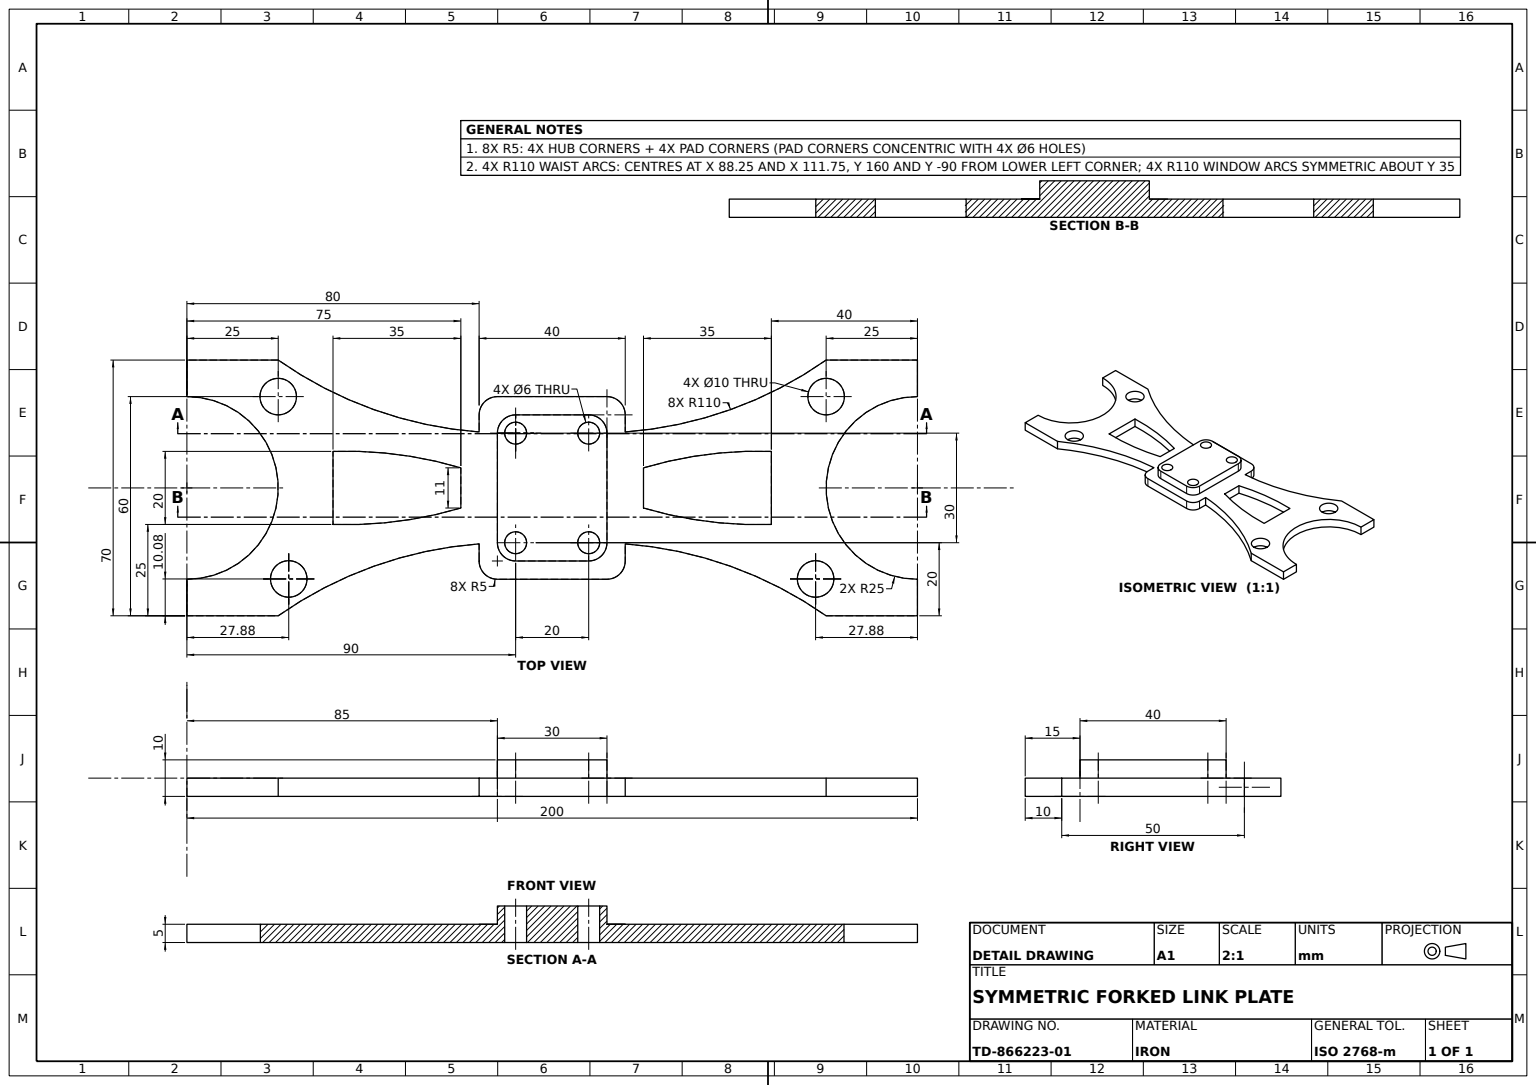
solid
v1 (100,35,-5)
v2 (75,35,-5)
e1 v1 v2 LINE
v3 (75,35,0)
e2 v3 v2 LINE
v4 (100,35,0)
e3 v4 v3 LINE
e4 v4 v1 LINE
face PLANE(AX(P(-100,35,0),D(0,1,0),D(1,0,0))) [e1 -e2 -e3 e4]
v5 (-20,15.309477,0)
v6 (-20,20,0)
e5 v5 v6 LINE
v7 (-20,20,-5)
e6 v6 v7 LINE
v8 (-20,15.309477,-5)
e7 v8 v7 LINE
e8 v5 v8 LINE
face PLANE(AX(P(-20,15.309477,0),D(-1,0,0),D(0,1,0))) [e5 e6 -e7 -e8]
v9 (20,20,-5)
v10 (20,15.309477,-5)
e9 v9 v10 LINE
v11 (20,20,0)
e10 v11 v9 LINE
v12 (20,15.309477,0)
e11 v11 v12 LINE
e12 v12 v10 LINE
face PLANE(AX(P(20,-15.309477,0),D(1,0,0),D(0,-1,0))) [-e9 -e10 e11 e12]
v13 (-15,-15,0)
v14 (-15,15,0)
e13 v13 v14 LINE
v15 (-15,-15,5)
e14 v13 v15 LINE
v16 (-15,15,5)
e15 v15 v16 LINE
e16 v14 v16 LINE
face PLANE(AX(P(-15,-20,0),D(1,0,0),D(0,1,0))) rev [-e13 e14 e15 -e16]
v17 (-100,-25,0)
v18 (-100,-35,0)
e17 v17 v18 LINE
v19 (-100,-25,-5)
e18 v17 v19 LINE
v20 (-100,-35,-5)
e19 v19 v20 LINE
e20 v18 v20 LINE
face PLANE(AX(P(-100,25,0),D(-1,0,0),D(0,1,0))) [-e17 e18 e19 -e20]
v21 (-20,-15.309477,-5)
v22 (-75,-35,-5)
e21 v21 v22 CIRCLE(AX(P(-11.754447,-125,-5),D(0,0,1),D(1,0,0)),110)
v23 (-20,-15.309477,0)
e22 v23 v21 LINE
v24 (-75,-35,0)
e23 v23 v24 CIRCLE(AX(P(-11.754447,-125,0),D(0,0,1),D(1,0,0)),110)
e24 v24 v22 LINE
face CYL(AX(P(-11.754447,-125,-2.5),D(0,0,1),D(1,0,0)),110) rev [-e21 -e22 e23 e24]
v25 (15,-25,-5)
v26 (-15,-25,-5)
e25 v25 v26 LINE
v27 (15,-25,0)
e26 v27 v25 LINE
v28 (-15,-25,0)
e27 v27 v28 LINE
e28 v28 v26 LINE
face PLANE(AX(P(20,-25,0),D(0,-1,0),D(-1,0,0))) [-e25 -e26 e27 e28]
v29 (75,-35,0)
v30 (75,-35,-5)
e29 v29 v30 LINE
v31 (20,-15.309477,0)
e30 v29 v31 CIRCLE(AX(P(11.754447,-125,0),D(0,0,1),D(1,0,0)),110)
v32 (20,-15.309477,-5)
e31 v31 v32 LINE
e32 v30 v32 CIRCLE(AX(P(11.754447,-125,-5),D(0,0,1),D(1,0,0)),110)
face CYL(AX(P(11.754447,-125,-2.5),D(0,0,1),D(1,0,0)),110) rev [-e29 e30 e31 -e32]
v33 (-10,-20,0)
v34 (-10,-20,5)
e33 v33 v34 LINE
e34 v15 v34 CIRCLE(AX(P(-10,-15,5),D(0,0,1),D(1,0,0)),5)
e35 v13 v33 CIRCLE(AX(P(-10,-15,0),D(0,0,1),D(1,0,0)),5)
face CYL(AX(P(-10,-15,2.5),D(0,0,1),D(0,-1,0)),5) [e33 -e34 -e14 e35]
v35 (60,10,-5)
v36 (25,5.5,-5)
e36 v35 v36 CIRCLE(AX(P(56.345765,-99.939286,-5),D(0,0,1),D(1,0,0)),110)
v37 (60,10,0)
e37 v37 v35 LINE
v38 (25,5.5,0)
e38 v37 v38 CIRCLE(AX(P(56.345765,-99.939286,0),D(0,0,1),D(1,0,0)),110)
e39 v38 v36 LINE
face CYL(AX(P(56.345765,-99.939286,-2.5),D(0,0,1),D(1,0,0)),110) rev [-e36 -e37 e38 e39]
e40 v20 v22 LINE
e41 v18 v24 LINE
face PLANE(AX(P(-100,-35,0),D(0,1,0),D(1,0,0))) rev [e20 e40 -e24 -e41]
v39 (-70,25,0)
e42 v39 v39 CIRCLE(AX(P(-75,25,0),D(0,0,1),D(1,0,0)),5)
v40 (-70,25,-5)
e43 v40 v40 CIRCLE(AX(P(-75,25,-5),D(0,0,1),D(1,0,0)),5)
face CYL(AX(P(-75,25,-2.5),D(0,0,1),D(1,0,0)),5) rev [e42] [-e43]
v41 (-20,-20,-5)
e44 v41 v21 LINE
v42 (-20,-20,0)
e45 v42 v41 LINE
e46 v42 v23 LINE
face PLANE(AX(P(-20,15.309477,0),D(-1,0,0),D(0,1,0))) [e22 -e44 -e45 e46]
v43 (80,25,-5)
e47 v43 v43 CIRCLE(AX(P(75,25,-5),D(0,0,1),D(1,0,0)),5)
v44 (80,25,0)
e48 v44 v44 CIRCLE(AX(P(75,25,0),D(0,0,1),D(1,0,0)),5)
face CYL(AX(P(75,25,-2.5),D(0,0,1),D(1,0,0)),5) rev [-e47] [e48]
e49 v41 v26 CIRCLE(AX(P(-15,-20,-5),D(0,0,1),D(1,0,0)),5)
e50 v42 v28 CIRCLE(AX(P(-15,-20,0),D(0,0,1),D(1,0,0)),5)
face CYL(AX(P(-15,-20,-2.5),D(0,0,-1),D(-1,0,0)),5) [e45 e49 -e28 -e50]
v45 (13,15,5)
e51 v45 v45 CIRCLE(AX(P(10,15,5),D(0,0,1),D(1,0,0)),3)
v46 (13,15,-5)
e52 v46 v46 CIRCLE(AX(P(10,15,-5),D(0,0,1),D(1,0,0)),3)
face CYL(AX(P(10,15,-10),D(0,0,1),D(1,0,0)),3) rev [e51] [-e52]
v47 (15,25,-5)
e53 v9 v47 CIRCLE(AX(P(15,20,-5),D(0,0,1),D(1,0,0)),5)
v48 (15,25,0)
e54 v48 v47 LINE
e55 v11 v48 CIRCLE(AX(P(15,20,0),D(0,0,1),D(1,0,0)),5)
face CYL(AX(P(15,20,-2.5),D(0,0,-1),D(1,0,0)),5) [e10 e53 -e54 -e55]
v49 (-60,-10,-5)
v50 (-25,-5.5,-5)
e56 v49 v50 CIRCLE(AX(P(-56.345765,99.939286,-5),D(0,0,1),D(1,0,0)),110)
v51 (-60,-10,0)
e57 v51 v49 LINE
v52 (-25,-5.5,0)
e58 v51 v52 CIRCLE(AX(P(-56.345765,99.939286,0),D(0,0,1),D(1,0,0)),110)
e59 v52 v50 LINE
face CYL(AX(P(-56.345765,99.939286,-2.5),D(0,0,1),D(1,0,0)),110) rev [-e56 -e57 e58 e59]
v53 (100,25,0)
e60 v53 v4 LINE
v54 (100,25,-5)
e61 v53 v54 LINE
e62 v54 v1 LINE
face PLANE(AX(P(100,-25,0),D(1,0,0),D(0,-1,0))) [-e4 -e60 e61 e62]
v55 (100,-35,-5)
e63 v55 v30 LINE
v56 (100,-35,0)
e64 v56 v55 LINE
e65 v56 v29 LINE
face PLANE(AX(P(-100,-35,0),D(0,1,0),D(1,0,0))) rev [e29 -e63 -e64 e65]
v57 (60,-10,0)
v58 (60,-10,-5)
e66 v57 v58 LINE
e67 v57 v37 LINE
e68 v58 v35 LINE
face PLANE(AX(P(60,-10,0),D(-1,0,0),D(0,1,0))) [-e66 e67 e37 -e68]
v59 (-7,15.000214,5)
e69 v59 v59 CIRCLE(AX(P(-10,15.000214,5),D(0,0,1),D(1,0,0)),3)
v60 (-7,15.000214,-5)
e70 v60 v60 CIRCLE(AX(P(-10,15.000214,-5),D(0,0,1),D(1,0,0)),3)
face CYL(AX(P(-10,15.000214,-10),D(0,0,1),D(1,0,0)),3) rev [e69] [-e70]
v61 (-100,25,0)
v62 (-100,25,-5)
e71 v61 v62 LINE
e72 v19 v62 CIRCLE(AX(P(-100,0,-5),D(0,0,1),D(1,0,0)),25)
e73 v17 v61 CIRCLE(AX(P(-100,0,0),D(0,0,1),D(1,0,0)),25)
face CYL(AX(P(-100,0,-2.5),D(0,0,1),D(1,0,0)),25) rev [e71 -e72 -e18 e73]
v63 (100,-25,0)
e74 v53 v63 CIRCLE(AX(P(100,0,0),D(0,0,1),D(1,0,0)),25)
v64 (100,-25,-5)
e75 v63 v64 LINE
e76 v54 v64 CIRCLE(AX(P(100,0,-5),D(0,0,1),D(1,0,0)),25)
face CYL(AX(P(100,0,-2.5),D(0,0,1),D(1,0,0)),25) rev [-e61 e74 e75 -e76]
v65 (-100,35,0)
e77 v61 v65 LINE
v66 (-100,35,-5)
e78 v65 v66 LINE
e79 v62 v66 LINE
face PLANE(AX(P(-100,25,0),D(-1,0,0),D(0,1,0))) [-e71 e77 e78 -e79]
v67 (-75,35,0)
e80 v65 v67 LINE
v68 (-75,35,-5)
e81 v67 v68 LINE
e82 v66 v68 LINE
face PLANE(AX(P(-100,35,0),D(0,1,0),D(1,0,0))) [-e78 e80 e81 -e82]
v69 (-15,25,-5)
e83 v69 v47 LINE
v70 (-15,25,0)
e84 v70 v69 LINE
e85 v70 v48 LINE
face PLANE(AX(P(-20,25,0),D(0,1,0),D(1,0,0))) [e54 -e83 -e84 e85]
e86 v12 v3 CIRCLE(AX(P(11.754447,125,0),D(0,0,1),D(1,0,0)),110)
e87 v10 v2 CIRCLE(AX(P(11.754447,125,-5),D(0,0,1),D(1,0,0)),110)
face CYL(AX(P(11.754447,125,-2.5),D(0,0,1),D(1,0,0)),110) rev [e86 e2 -e87 -e12]
v71 (20,-20,0)
e88 v31 v71 LINE
v72 (20,-20,-5)
e89 v71 v72 LINE
e90 v32 v72 LINE
face PLANE(AX(P(20,-15.309477,0),D(1,0,0),D(0,-1,0))) [-e31 e88 e89 -e90]
e91 v63 v56 LINE
e92 v64 v55 LINE
face PLANE(AX(P(100,-25,0),D(1,0,0),D(0,-1,0))) [e91 e64 -e92 -e75]
v73 (25,-5.5,0)
e93 v73 v57 CIRCLE(AX(P(56.345765,99.939286,0),D(0,0,1),D(1,0,0)),110)
e94 v73 v38 LINE
v74 (-67.116157,-24.916765,0)
e95 v74 v74 CIRCLE(AX(P(-72.116157,-24.916765,0),D(0,0,1),D(1,0,0)),5)
e96 v70 v6 CIRCLE(AX(P(-15,20,0),D(0,0,1),D(1,0,0)),5)
e97 v67 v5 CIRCLE(AX(P(-11.754447,125,0),D(0,0,1),D(1,0,0)),110)
e98 v27 v71 CIRCLE(AX(P(15,-20,0),D(0,0,1),D(1,0,0)),5)
v75 (10,-20,0)
v76 (15,-15,0)
e99 v75 v76 CIRCLE(AX(P(10,-15,0),D(0,0,1),D(1,0,0)),5)
e100 v75 v33 LINE
v77 (-10,20,0)
e101 v77 v14 CIRCLE(AX(P(-10,15,0),D(0,0,1),D(1,0,0)),5)
v78 (10,20,0)
e102 v77 v78 LINE
v79 (15,15,0)
e103 v79 v78 CIRCLE(AX(P(10,15,0),D(0,0,1),D(1,0,0)),5)
e104 v79 v76 LINE
v80 (-25,5.5,0)
e105 v52 v80 LINE
v81 (-60,10,0)
e106 v51 v81 LINE
e107 v80 v81 CIRCLE(AX(P(-56.345765,-99.939286,0),D(0,0,1),D(1,0,0)),110)
v82 (77.116157,-24.916765,0)
e108 v82 v82 CIRCLE(AX(P(72.116157,-24.916765,0),D(0,0,1),D(1,0,0)),5)
face PLANE(AX(P(0,0,0),D(0,0,1),D(1,0,0))) [-e48] [-e93 e94 -e38 -e67] [-e42] [-e95] [-e88 -e30 -e65 -e91 -e74 e60 e3 -e86 -e11 e55 -e85 e96 -e5 -e97 -e80 -e77 -e73 e17 e41 -e23 -e46 e50 -e27 e98] [-e99 e100 -e35 e13 -e101 e102 -e103 e104] [-e105 -e58 e106 -e107] [-e108]
v83 (-67.116157,-24.916765,-5)
e109 v83 v83 CIRCLE(AX(P(-72.116157,-24.916765,-5),D(0,0,1),D(1,0,0)),5)
face CYL(AX(P(-72.116157,-24.916765,-2.5),D(0,0,1),D(1,0,0)),5) rev [e95] [-e109]
v84 (-7,-15,-5)
e110 v84 v84 CIRCLE(AX(P(-10,-15,-5),D(0,0,1),D(1,0,0)),3)
v85 (-25,5.5,-5)
v86 (-60,10,-5)
e111 v85 v86 CIRCLE(AX(P(-56.345765,-99.939286,-5),D(0,0,1),D(1,0,0)),110)
e112 v49 v86 LINE
e113 v50 v85 LINE
v87 (25,-5.5,-5)
e114 v87 v58 CIRCLE(AX(P(56.345765,99.939286,-5),D(0,0,1),D(1,0,0)),110)
e115 v87 v36 LINE
e116 v68 v8 CIRCLE(AX(P(-11.754447,125,-5),D(0,0,1),D(1,0,0)),110)
e117 v69 v7 CIRCLE(AX(P(-15,20,-5),D(0,0,1),D(1,0,0)),5)
e118 v25 v72 CIRCLE(AX(P(15,-20,-5),D(0,0,1),D(1,0,0)),5)
v88 (13,-15,-5)
e119 v88 v88 CIRCLE(AX(P(10,-15,-5),D(0,0,1),D(1,0,0)),3)
v89 (77.116157,-24.916765,-5)
e120 v89 v89 CIRCLE(AX(P(72.116157,-24.916765,-5),D(0,0,1),D(1,0,0)),5)
face PLANE(AX(P(0,0,-5),D(0,0,1),D(1,0,0))) rev [e43] [e47] [e52] [e110] [e111 -e112 e56 e113] [e70] [e114 e68 e36 -e115] [e79 e82 e116 e7 -e117 e83 -e53 e9 e87 -e1 -e62 e76 e92 e63 e32 e90 -e118 e25 -e49 e44 e21 -e40 -e19 e72] [e119] [e120] [e109]
face CYL(AX(P(-11.754447,125,-2.5),D(0,0,1),D(1,0,0)),110) rev [-e116 -e81 e97 e8]
face CYL(AX(P(-15,20,-2.5),D(0,0,-1),D(0,1,0)),5) [-e6 -e96 e84 e117]
v90 (13,-15,5)
e121 v90 v90 CIRCLE(AX(P(10,-15,5),D(0,0,1),D(1,0,0)),3)
face CYL(AX(P(10,-15,2.5),D(0,0,1),D(1,0,0)),3) rev [e121] [-e119]
e122 v73 v87 LINE
face CYL(AX(P(56.345765,99.939286,-2.5),D(0,0,1),D(1,0,0)),110) rev [e93 e66 -e114 -e122]
v91 (-7,-15,5)
e123 v91 v91 CIRCLE(AX(P(-10,-15,5),D(0,0,1),D(1,0,0)),3)
face CYL(AX(P(-10,-15,2.5),D(0,0,1),D(1,0,0)),3) rev [-e110] [e123]
face CYL(AX(P(72.116157,-24.916765,-2.5),D(0,0,1),D(1,0,0)),5) rev [-e120] [e108]
e124 v81 v86 LINE
face PLANE(AX(P(-60,-10,0),D(-1,0,0),D(0,1,0))) rev [-e106 e57 e112 -e124]
v92 (-10,20,5)
e125 v92 v16 CIRCLE(AX(P(-10,15,5),D(0,0,1),D(1,0,0)),5)
e126 v77 v92 LINE
face CYL(AX(P(-10,15,2.5),D(0,0,1),D(-1,0,0)),5) [e101 e16 -e125 -e126]
v93 (15,-15,5)
e127 v76 v93 LINE
v94 (10,-20,5)
e128 v94 v93 CIRCLE(AX(P(10,-15,5),D(0,0,1),D(1,0,0)),5)
e129 v75 v94 LINE
face CYL(AX(P(10,-15,2.5),D(0,0,1),D(1,0,0)),5) [e127 -e128 -e129 e99]
e130 v80 v85 LINE
face PLANE(AX(P(-25,-5.5,0),D(-1,0,0),D(0,1,0))) [e130 -e113 -e59 e105]
face CYL(AX(P(-56.345765,-99.939286,-2.5),D(0,0,1),D(1,0,0)),110) rev [-e111 -e130 e107 e124]
face CYL(AX(P(15,-20,-2.5),D(0,0,-1),D(0,-1,0)),5) [e118 -e89 -e98 e26]
e131 v94 v34 LINE
face PLANE(AX(P(15,-20,0),D(0,1,0),D(-1,0,0))) rev [e129 e131 -e33 -e100]
v95 (10,20,5)
e132 v78 v95 LINE
e133 v92 v95 LINE
face PLANE(AX(P(-15,20,0),D(0,-1,0),D(1,0,0))) rev [-e132 -e102 e126 e133]
v96 (15,15,5)
e134 v79 v96 LINE
e135 v96 v93 LINE
face PLANE(AX(P(15,20,0),D(-1,0,0),D(0,-1,0))) rev [-e104 e134 e135 -e127]
face PLANE(AX(P(25,-5.5,0),D(-1,0,0),D(0,1,0))) rev [-e94 e122 e115 -e39]
e136 v96 v95 CIRCLE(AX(P(10,15,5),D(0,0,1),D(1,0,0)),5)
face PLANE(AX(P(0,0,5),D(0,0,1),D(1,0,0))) [-e123] [-e51] [-e135 e136 -e133 e125 -e15 e34 -e131 e128] [-e69] [-e121]
face CYL(AX(P(10,15,2.5),D(0,0,1),D(0,1,0)),5) [e132 -e136 -e134 e103]
